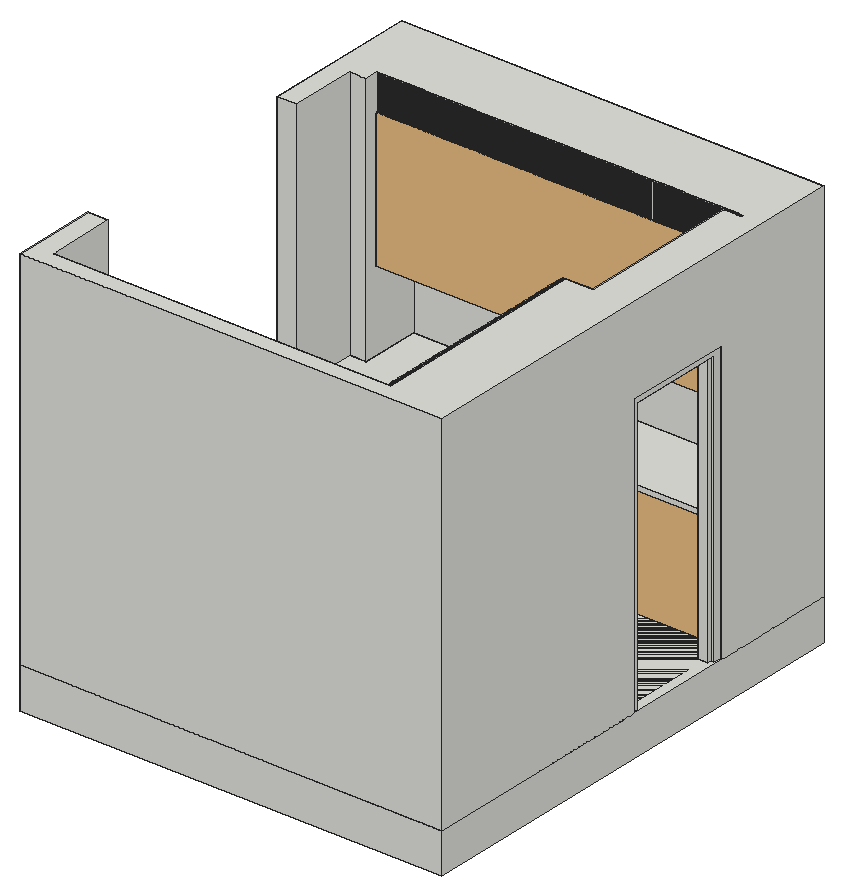
# SketchUp Ruby script. Lengths in millimetres.
U = 1.mm
M = Sketchup.active_model
def pt(a) = Geom::Point3d.new(a.map { |v| v * U })
def face(e, loops, mat)
  f = e.add_face(loops[0].map { |a| pt(a) })
  loops[1..].each { |l| e.add_face(l.map { |a| pt(a) }).erase! }
  f.material = f.back_material = mat if mat
  f
end
# faces: each face lists its corners as indices into pts; further lists are holes
def faces(e, pts, list, mat = nil) = list.each { |f| face(e, (f[0].is_a?(Array) ? f : [f]).map { |l| l.map { |i| pts[i] } }, mat) }
# xy, xz, yz: faces in a plane at the given z, y or x. An outline is a flat list of corners, or four numbers for a rectangle; further outlines are holes
def ring(l) = l.size == 4 ? [[l[0], l[1]], [l[2], l[1]], [l[2], l[3]], [l[0], l[3]]] : l.each_slice(2).to_a
def flat(e, list, mat, &to3) = list.each { |f| face(e, (f[0].is_a?(Array) ? f : [f]).map { |l| ring(l).map { |u, v| to3.(u, v) } }, mat) }
def xy(e, z, list, mat = nil) = flat(e, list, mat) { |x, y| [x, y, z] }
def xz(e, y, list, mat = nil) = flat(e, list, mat) { |x, z| [x, y, z] }
def yz(e, x, list, mat = nil) = flat(e, list, mat) { |y, z| [x, y, z] }
def lines(e, pts, list) = list.each { |a, b| e.add_line(pt(pts[a]), pt(pts[b])) }
# prism: a flat outline (further loops are holes) pulled along v
def prism(e, loops, v, mat = nil)
  f = face(e, loops, mat); d = Geom::Vector3d.new(v.map { |x| x * U })
  f.pushpull(f.normal.samedirection?(d) ? d.length : -d.length)
end
def box(e, o, s, mat = nil) = prism(e, [[o, [o[0] + s[0], o[1], o[2]], [o[0] + s[0], o[1] + s[1], o[2]], [o[0], o[1] + s[1], o[2]]]], [0, 0, s[2]], mat)
def at(x, y, z, deg = 0) = Geom::Transformation.translation(pt([x, y, z])) * Geom::Transformation.rotation(ORIGIN, Z_AXIS, deg.degrees)
def axes(o, x, y, z) = Geom::Transformation.new([*x, 0, *y, 0, *z, 0, *pt(o).to_a, 1])
def part(name) = M.definitions.add(name)
# library, detail: a bought-in or finely detailed component or shape, given as its bounding box
def library(name, o, s) = part(name).tap { |d| box(d.entities, o, s) }
def detail(e, o, s) = box(e.add_group.entities, o, s)
def put(e, d, t, mat = nil) = e.add_instance(d, t).tap { |i| i.material = mat if mat }
def group(e, t, mat = nil) = e.add_group.tap { |g| g.transformation = t; g.material = mat if mat }.entities
root = M.entities
c1 = part("skp9A08")
detail(c1.entities,[955.4,-577.1,1130.3],[195.9,193,77.6])
c2 = part("Memento Mori 2 - Living Room and Bedroom JhonyHebert")
put(c2.entities,c1,at(1865.8,0,3866.9))
c3 = part("Basket")
put(c3.entities,c2,at(22136,105695.5,0))
c4 = library("Group\#3",[-125,0,0],[2845,600,820])
c5 = library("Group\#4",[0,-350,0],[2720,368,1030])
c6 = part("Group5\#1")
xy(c6.entities,0,[[-410,-1050,-410,1050,410,1050,410,-1050,360,-1050,360,1000,-360,1000,-360,-1050]])
xy(c6.entities,25,[[-360,-1050,-360,1000,360,1000,360,-1050,335,-1050,335,975,-335,975,-335,-1050]])
xy(c6.entities,100,[[-360,-1050,-335,-1050,-335,975,335,975,335,-1050,360,-1050,360,1000,-360,1000]])
xy(c6.entities,125,[[-410,-1050,-360,-1050,-360,1000,360,1000,360,-1050,410,-1050,410,1050,-410,1050]])
xz(c6.entities,-1050,[[-410,0,-360,125],[360,0,410,125],[-360,25,-335,100],[335,25,360,100]])
xz(c6.entities,975,[[-335,25,335,100]])
xz(c6.entities,1000,[[-360,0,360,25],[-360,100,360,125]])
xz(c6.entities,1050,[[-410,0,410,125]])
yz(c6.entities,-410,[[-1050,0,1050,125]])
yz(c6.entities,-360,[[-1050,0,1000,25],[-1050,100,1000,125]])
yz(c6.entities,-335,[[-1050,25,975,100]])
yz(c6.entities,335,[[-1050,25,975,100]])
yz(c6.entities,360,[[-1050,0,1000,25],[-1050,100,1000,125]])
yz(c6.entities,410,[[-1050,0,1050,125]])
c7 = library("Group\#5",[-350,0,0],[350,1630,1030])
c8 = part("Group\#6")
box(c8.entities,[-20,0,0],[20,15.2,260])
xy(root,0,[[0,0,0,634,148,634,148,124,2993,124,2993,1784,3148,1784,3148,0],[148,124,2993,124,2993,1784,3070.5,1784,3070.5,2604,2993,2604,2993,3324,273,3324,273,2884,148,2884,148,2394,0,2394,0,634,148,634],[3070.5,1784,3148,2604],[0,2394,0,3553,3148,3553,3148,2604,2993,2604,2993,3324,273,3324,273,2884,148,2884,148,2394]])
xy(root,100,[[2393,124,2993,724],[2393,724,2993,774],[2393,774,2993,1304],[2393,1304,2993,1754]])
xy(root,125,[[2393,1329,2993,1729]])
xy(root,451,[[2393,124,2411,724],[2393,774,2411,1304]])
xy(root,469,[[2393,124,2411,724],[2393,774,2411,1304]])
xy(root,790,[[2393,124,2993,724],[2393,774,2411,1304]])
xy(root,795,[[2393,1329,2993,1729]])
xy(root,820,[[2393,724,2993,774],[2411,774,2993,1304],[2393,1304,2993,1754]])
xy(root,2100,[[2993,1784,3070.5,2604],[3070.5,1784,3148,2604]])
xy(root,2490,[[2663,124,2993,1754],[288,2974,303,2986],[308,2974,323,2986],[328,2974,343,2986],[348,2974,363,2986],
  [368,2974,383,2986],[388,2974,403,2986],[408,2974,423,2986],[428,2974,443,2986],[448,2974,463,2986],
  [468,2974,483,2986],[488,2974,503,2986],[508,2974,523,2986],[528,2974,543,2986],[548,2974,563,2986],
  [568,2974,583,2986],[588,2974,603,2986],[608,2974,623,2986],[628,2974,643,2986],[648,2974,663,2986],
  [668,2974,683,2986],[688,2974,703,2986],[708,2974,723,2986],[728,2974,743,2986],[748,2974,763,2986],
  [768,2974,783,2986],[788,2974,803,2986],[808,2974,823,2986],[828,2974,843,2986],[848,2974,863,2986],
  [868,2974,883,2986],[888,2974,903,2986],[908,2974,923,2986],[928,2974,943,2986],[948,2974,963,2986],
  [968,2974,983,2986],[988,2974,1003,2986],[1008,2974,1023,2986],[1028,2974,1043,2986],[1048,2974,1063,2986],
  [1068,2974,1083,2986],[1088,2974,1103,2986],[1108,2974,1123,2986],[1128,2974,1143,2986],[1148,2974,1163,2986],
  [1168,2974,1183,2986],[1188,2974,1203,2986],[1208,2974,1223,2986],[1228,2974,1243,2986],[1248,2974,1263,2986],
  [1268,2974,1283,2986],[1288,2974,1303,2986],[1308,2974,1323,2986],[1328,2974,1343,2986],[1348,2974,1363,2986],
  [1368,2974,1383,2986],[1388,2974,1403,2986],[1408,2974,1423,2986],[1428,2974,1443,2986],[1448,2974,1463,2986],
  [1468,2974,1483,2986],[1488,2974,1503,2986],[1508,2974,1523,2986],[1528,2974,1543,2986],[1548,2974,1563,2986],
  [1568,2974,1583,2986],[1588,2974,1603,2986],[1608,2974,1623,2986],[1628,2974,1643,2986],[1648,2974,1663,2986],
  [1668,2974,1683,2986],[1688,2974,1703,2986],[1708,2974,1723,2986],[1728,2974,1743,2986],[1748,2974,1763,2986],
  [1768,2974,1783,2986],[1788,2974,1803,2986],[1808,2974,1823,2986],[1828,2974,1843,2986],[1848,2974,1863,2986],
  [1868,2974,1883,2986],[1888,2974,1903,2986],[1908,2974,1923,2986],[1928,2974,1943,2986],[1948,2974,1963,2986],
  [1968,2974,1983,2986],[1988,2974,2003,2986],[2008,2974,2023,2986],[2028,2974,2043,2986],[2048,2974,2063,2986],
  [2068,2974,2083,2986],[2088,2974,2103,2986],[2108,2974,2123,2986],[2128,2974,2143,2986],[2148,2974,2163,2986],
  [2168,2974,2183,2986],[2188,2974,2203,2986],[2208,2974,2223,2986],[2228,2974,2243,2986],[2248,2974,2263,2986],
  [2268,2974,2283,2986],[2288,2974,2303,2986],[2308,2974,2323,2986],[2328,2974,2343,2986],[2348,2974,2363,2986],
  [2368,2974,2383,2986],[2388,2974,2403,2986],[2408,2974,2423,2986],[2428,2974,2443,2986],[2448,2974,2463,2986],
  [2468,2974,2483,2986],[2488,2974,2503,2986],[2508,2974,2523,2986],[2528,2974,2543,2986],[2548,2974,2563,2986],
  [2568,2974,2583,2986],[2588,2974,2603,2986],[2608,2974,2623,2986],[2628,2974,2643,2986],[2648,2974,2663,2986],
  [2668,2974,2683,2986],[2688,2974,2703,2986],[2708,2974,2723,2986],[2728,2974,2743,2986],[2748,2974,2763,2986],
  [2768,2974,2783,2986],[2788,2974,2803,2986],[2808,2974,2823,2986],[2828,2974,2843,2986],[2848,2974,2863,2986],
  [2868,2974,2883,2986],[2888,2974,2903,2986],[2908,2974,2923,2986],[2928,2974,2943,2986],[2948,2974,2963,2986],
  [2968,2974,2983,2986],[2988,2974,3003,2986],[273,2986,309.5,3324],[309.5,2986,316.5,3324],[316.5,2986,1149.5,3324],
  [1149.5,2986,1156.5,3324],[1156.5,2986,1729.5,3324],[1729.5,2986,2376.5,3324],[2376.5,2986,2949.5,3324],[2949.5,2986,2956.5,3324],
  [2956.5,2986,2993,3324]])
xy(root,2600,[[2868,1754,2993,2986]])
xy(root,2750,[[[0,0,3148,0,3148,3553,0,3553,0,2394,148,2394,148,2884,273,2884,273,2986,2883,2986,2883,2974,2868,2974,2868,1754,2663,1754,2663,124,148,124,148,634,0,634],[2908,2974,2923,2986],[2928,2974,2943,2986],[2988,2974,3003,2986],[2968,2974,2983,2986],[2888,2974,2903,2986],[2948,2974,2963,2986]],[288,2974,303,2986],[308,2974,323,2986],[328,2974,343,2986],[348,2974,363,2986],
  [368,2974,383,2986],[388,2974,403,2986],[408,2974,423,2986],[428,2974,443,2986],[448,2974,463,2986],
  [468,2974,483,2986],[488,2974,503,2986],[508,2974,523,2986],[528,2974,543,2986],[548,2974,563,2986],
  [568,2974,583,2986],[588,2974,603,2986],[608,2974,623,2986],[628,2974,643,2986],[648,2974,663,2986],
  [668,2974,683,2986],[688,2974,703,2986],[708,2974,723,2986],[728,2974,743,2986],[748,2974,763,2986],
  [768,2974,783,2986],[788,2974,803,2986],[808,2974,823,2986],[828,2974,843,2986],[848,2974,863,2986],
  [868,2974,883,2986],[888,2974,903,2986],[908,2974,923,2986],[928,2974,943,2986],[948,2974,963,2986],
  [968,2974,983,2986],[988,2974,1003,2986],[1008,2974,1023,2986],[1028,2974,1043,2986],[1048,2974,1063,2986],
  [1068,2974,1083,2986],[1088,2974,1103,2986],[1108,2974,1123,2986],[1128,2974,1143,2986],[1148,2974,1163,2986],
  [1168,2974,1183,2986],[1188,2974,1203,2986],[1208,2974,1223,2986],[1228,2974,1243,2986],[1248,2974,1263,2986],
  [1268,2974,1283,2986],[1288,2974,1303,2986],[1308,2974,1323,2986],[1328,2974,1343,2986],[1348,2974,1363,2986],
  [1368,2974,1383,2986],[1388,2974,1403,2986],[1408,2974,1423,2986],[1428,2974,1443,2986],[1448,2974,1463,2986],
  [1468,2974,1483,2986],[1488,2974,1503,2986],[1508,2974,1523,2986],[1528,2974,1543,2986],[1548,2974,1563,2986],
  [1568,2974,1583,2986],[1588,2974,1603,2986],[1608,2974,1623,2986],[1628,2974,1643,2986],[1648,2974,1663,2986],
  [1668,2974,1683,2986],[1688,2974,1703,2986],[1708,2974,1723,2986],[1728,2974,1743,2986],[1748,2974,1763,2986],
  [1768,2974,1783,2986],[1788,2974,1803,2986],[1808,2974,1823,2986],[1828,2974,1843,2986],[1848,2974,1863,2986],
  [1868,2974,1883,2986],[1888,2974,1903,2986],[1908,2974,1923,2986],[1928,2974,1943,2986],[1948,2974,1963,2986],
  [1968,2974,1983,2986],[1988,2974,2003,2986],[2008,2974,2023,2986],[2028,2974,2043,2986],[2048,2974,2063,2986],
  [2068,2974,2083,2986],[2088,2974,2103,2986],[2108,2974,2123,2986],[2128,2974,2143,2986],[2148,2974,2163,2986],
  [2168,2974,2183,2986],[2188,2974,2203,2986],[2208,2974,2223,2986],[2228,2974,2243,2986],[2248,2974,2263,2986],
  [2268,2974,2283,2986],[2288,2974,2303,2986],[2308,2974,2323,2986],[2328,2974,2343,2986],[2348,2974,2363,2986],
  [2368,2974,2383,2986],[2388,2974,2403,2986],[2408,2974,2423,2986],[2428,2974,2443,2986],[2448,2974,2463,2986],
  [2468,2974,2483,2986],[2488,2974,2503,2986],[2508,2974,2523,2986],[2528,2974,2543,2986],[2548,2974,2563,2986],
  [2568,2974,2583,2986],[2588,2974,2603,2986],[2608,2974,2623,2986],[2628,2974,2643,2986],[2648,2974,2663,2986],
  [2668,2974,2683,2986],[2688,2974,2703,2986],[2708,2974,2723,2986],[2728,2974,2743,2986],[2748,2974,2763,2986],
  [2768,2974,2783,2986],[2788,2974,2803,2986],[2808,2974,2823,2986],[2828,2974,2843,2986],[2848,2974,2863,2986],
  [2868,2974,2883,2986],[2888,2974,2903,2986],[2908,2974,2923,2986],[2928,2974,2943,2986],[2948,2974,2963,2986],
  [2968,2974,2983,2986],[2988,2974,3003,2986]])
xz(root,0,[[0,0,3148,2750]])
xz(root,124,[[148,0,148,2750,2663,2750,2663,2490,2993,2490,2993,790,2393,790,2393,469,2411,469,2411,451,2393,451,2393,100,2993,100,2993,0],[2393,100,2393,451,2411,451,2411,469,2393,469,2393,790,2993,790,2993,100]])
xz(root,634,[[0,0,148,2750]])
xz(root,724,[[2393,451,2411,469],[2393,790,2993,820]])
xz(root,774,[[2393,451,2411,469],[2393,790,2411,820]])
xz(root,1304,[[2393,451,2411,460],[2393,460,2411,469],[2393,790,2411,820]])
xz(root,1329,[[2393,125,2993,795]])
xz(root,1729,[[2393,125,2993,795]])
xz(root,1754,[[2393,100,2993,820],[2663,2490,2663,2750,2868,2750,2868,2600,2993,2600,2993,2490]])
xz(root,1784,[[2993,0,3070.5,2100],[3070.5,0,3148,2100]])
xz(root,2394,[[0,0,148,2750]])
xz(root,2604,[[2993,0,3070.5,2100],[3070.5,0,3148,2100]])
xz(root,2884,[[148,0,273,860],[148,860,273,2750]])
xz(root,2974,[[288,2490,303,2750],[308,2490,323,2750],[328,2490,343,2750],[348,2490,363,2750],[368,2490,383,2750],
  [388,2490,403,2750],[408,2490,423,2750],[428,2490,443,2750],[448,2490,463,2750],[468,2490,483,2750],
  [488,2490,503,2750],[508,2490,523,2750],[528,2490,543,2750],[548,2490,563,2750],[568,2490,583,2750],
  [588,2490,603,2750],[608,2490,623,2750],[628,2490,643,2750],[648,2490,663,2750],[668,2490,683,2750],
  [688,2490,703,2750],[708,2490,723,2750],[728,2490,743,2750],[748,2490,763,2750],[768,2490,783,2750],
  [788,2490,803,2750],[808,2490,823,2750],[828,2490,843,2750],[848,2490,863,2750],[868,2490,883,2750],
  [888,2490,903,2750],[908,2490,923,2750],[928,2490,943,2750],[948,2490,963,2750],[968,2490,983,2750],
  [988,2490,1003,2750],[1008,2490,1023,2750],[1028,2490,1043,2750],[1048,2490,1063,2750],[1068,2490,1083,2750],
  [1088,2490,1103,2750],[1108,2490,1123,2750],[1128,2490,1143,2750],[1148,2490,1163,2750],[1168,2490,1183,2750],
  [1188,2490,1203,2750],[1208,2490,1223,2750],[1228,2490,1243,2750],[1248,2490,1263,2750],[1268,2490,1283,2750],
  [1288,2490,1303,2750],[1308,2490,1323,2750],[1328,2490,1343,2750],[1348,2490,1363,2750],[1368,2490,1383,2750],
  [1388,2490,1403,2750],[1408,2490,1423,2750],[1428,2490,1443,2750],[1448,2490,1463,2750],[1468,2490,1483,2750],
  [1488,2490,1503,2750],[1508,2490,1523,2750],[1528,2490,1543,2750],[1548,2490,1563,2750],[1568,2490,1583,2750],
  [1588,2490,1603,2750],[1608,2490,1623,2750],[1628,2490,1643,2750],[1648,2490,1663,2750],[1668,2490,1683,2750],
  [1688,2490,1703,2750],[1708,2490,1723,2750],[1728,2490,1743,2750],[1748,2490,1763,2750],[1768,2490,1783,2750],
  [1788,2490,1803,2750],[1808,2490,1823,2750],[1828,2490,1843,2750],[1848,2490,1863,2750],[1868,2490,1883,2750],
  [1888,2490,1903,2750],[1908,2490,1923,2750],[1928,2490,1943,2750],[1948,2490,1963,2750],[1968,2490,1983,2750],
  [1988,2490,2003,2750],[2008,2490,2023,2750],[2028,2490,2043,2750],[2048,2490,2063,2750],[2068,2490,2083,2750],
  [2088,2490,2103,2750],[2108,2490,2123,2750],[2128,2490,2143,2750],[2148,2490,2163,2750],[2168,2490,2183,2750],
  [2188,2490,2203,2750],[2208,2490,2223,2750],[2228,2490,2243,2750],[2248,2490,2263,2750],[2268,2490,2283,2750],
  [2288,2490,2303,2750],[2308,2490,2323,2750],[2328,2490,2343,2750],[2348,2490,2363,2750],[2368,2490,2383,2750],
  [2388,2490,2403,2750],[2408,2490,2423,2750],[2428,2490,2443,2750],[2448,2490,2463,2750],[2468,2490,2483,2750],
  [2488,2490,2503,2750],[2508,2490,2523,2750],[2528,2490,2543,2750],[2548,2490,2563,2750],[2568,2490,2583,2750],
  [2588,2490,2603,2750],[2608,2490,2623,2750],[2628,2490,2643,2750],[2648,2490,2663,2750],[2668,2490,2683,2750],
  [2688,2490,2703,2750],[2708,2490,2723,2750],[2728,2490,2743,2750],[2748,2490,2763,2750],[2768,2490,2783,2750],
  [2788,2490,2803,2750],[2808,2490,2823,2750],[2828,2490,2843,2750],[2848,2490,2863,2750],[2868,2490,2883,2750],
  [2888,2490,2903,2750],[2908,2490,2923,2750],[2928,2490,2943,2750],[2948,2490,2963,2750],[2968,2490,2983,2750],
  [2988,2490,3003,2750]])
xz(root,2986,[[273,2490,288,2750],[288,2490,303,2750],[303,2490,308,2750],[308,2490,323,2750],[323,2490,328,2750],
  [328,2490,343,2750],[343,2490,348,2750],[348,2490,363,2750],[363,2490,368,2750],[368,2490,383,2750],
  [383,2490,388,2750],[388,2490,403,2750],[403,2490,408,2750],[408,2490,423,2750],[423,2490,428,2750],
  [428,2490,443,2750],[443,2490,448,2750],[448,2490,463,2750],[463,2490,468,2750],[468,2490,483,2750],
  [483,2490,488,2750],[488,2490,503,2750],[503,2490,508,2750],[508,2490,523,2750],[523,2490,528,2750],
  [528,2490,543,2750],[543,2490,548,2750],[548,2490,563,2750],[563,2490,568,2750],[568,2490,583,2750],
  [583,2490,588,2750],[588,2490,603,2750],[603,2490,608,2750],[608,2490,623,2750],[623,2490,628,2750],
  [628,2490,643,2750],[643,2490,648,2750],[648,2490,663,2750],[663,2490,668,2750],[668,2490,683,2750],
  [683,2490,688,2750],[688,2490,703,2750],[703,2490,708,2750],[708,2490,723,2750],[723,2490,728,2750],
  [728,2490,743,2750],[743,2490,748,2750],[748,2490,763,2750],[763,2490,768,2750],[768,2490,783,2750],
  [783,2490,788,2750],[788,2490,803,2750],[803,2490,808,2750],[808,2490,823,2750],[823,2490,828,2750],
  [828,2490,843,2750],[843,2490,848,2750],[848,2490,863,2750],[863,2490,868,2750],[868,2490,883,2750],
  [883,2490,888,2750],[888,2490,903,2750],[903,2490,908,2750],[908,2490,923,2750],[923,2490,928,2750],
  [928,2490,943,2750],[943,2490,948,2750],[948,2490,963,2750],[963,2490,968,2750],[968,2490,983,2750],
  [983,2490,988,2750],[988,2490,1003,2750],[1003,2490,1008,2750],[1008,2490,1023,2750],[1023,2490,1028,2750],
  [1028,2490,1043,2750],[1043,2490,1048,2750],[1048,2490,1063,2750],[1063,2490,1068,2750],[1068,2490,1083,2750],
  [1083,2490,1088,2750],[1088,2490,1103,2750],[1103,2490,1108,2750],[1108,2490,1123,2750],[1123,2490,1128,2750],
  [1128,2490,1143,2750],[1143,2490,1148,2750],[1148,2490,1163,2750],[1163,2490,1168,2750],[1168,2490,1183,2750],
  [1183,2490,1188,2750],[1188,2490,1203,2750],[1203,2490,1208,2750],[1208,2490,1223,2750],[1223,2490,1228,2750],
  [1228,2490,1243,2750],[1243,2490,1248,2750],[1248,2490,1263,2750],[1263,2490,1268,2750],[1268,2490,1283,2750],
  [1283,2490,1288,2750],[1288,2490,1303,2750],[1303,2490,1308,2750],[1308,2490,1323,2750],[1323,2490,1328,2750],
  [1328,2490,1343,2750],[1343,2490,1348,2750],[1348,2490,1363,2750],[1363,2490,1368,2750],[1368,2490,1383,2750],
  [1383,2490,1388,2750],[1388,2490,1403,2750],[1403,2490,1408,2750],[1408,2490,1423,2750],[1423,2490,1428,2750],
  [1428,2490,1443,2750],[1443,2490,1448,2750],[1448,2490,1463,2750],[1463,2490,1468,2750],[1468,2490,1483,2750],
  [1483,2490,1488,2750],[1488,2490,1503,2750],[1503,2490,1508,2750],[1508,2490,1523,2750],[1523,2490,1528,2750],
  [1528,2490,1543,2750],[1543,2490,1548,2750],[1548,2490,1563,2750],[1563,2490,1568,2750],[1568,2490,1583,2750],
  [1583,2490,1588,2750],[1588,2490,1603,2750],[1603,2490,1608,2750],[1608,2490,1623,2750],[1623,2490,1628,2750],
  [1628,2490,1643,2750],[1643,2490,1648,2750],[1648,2490,1663,2750],[1663,2490,1668,2750],[1668,2490,1683,2750],
  [1683,2490,1688,2750],[1688,2490,1703,2750],[1703,2490,1708,2750],[1708,2490,1723,2750],[1723,2490,1728,2750],
  [1728,2490,1743,2750],[1743,2490,1748,2750],[1748,2490,1763,2750],[1763,2490,1768,2750],[1768,2490,1783,2750],
  [1783,2490,1788,2750],[1788,2490,1803,2750],[1803,2490,1808,2750],[1808,2490,1823,2750],[1823,2490,1828,2750],
  [1828,2490,1843,2750],[1843,2490,1848,2750],[1848,2490,1863,2750],[1863,2490,1868,2750],[1868,2490,1883,2750],
  [1883,2490,1888,2750],[1888,2490,1903,2750],[1903,2490,1908,2750],[1908,2490,1923,2750],[1923,2490,1928,2750],
  [1928,2490,1943,2750],[1943,2490,1948,2750],[1948,2490,1963,2750],[1963,2490,1968,2750],[1968,2490,1983,2750],
  [1983,2490,1988,2750],[1988,2490,2003,2750],[2003,2490,2008,2750],[2008,2490,2023,2750],[2023,2490,2028,2750],
  [2028,2490,2043,2750],[2043,2490,2048,2750],[2048,2490,2063,2750],[2063,2490,2068,2750],[2068,2490,2083,2750],
  [2083,2490,2088,2750],[2088,2490,2103,2750],[2103,2490,2108,2750],[2108,2490,2123,2750],[2123,2490,2128,2750],
  [2128,2490,2143,2750],[2143,2490,2148,2750],[2148,2490,2163,2750],[2163,2490,2168,2750],[2168,2490,2183,2750],
  [2183,2490,2188,2750],[2188,2490,2203,2750],[2203,2490,2208,2750],[2208,2490,2223,2750],[2223,2490,2228,2750],
  [2228,2490,2243,2750],[2243,2490,2248,2750],[2248,2490,2263,2750],[2263,2490,2268,2750],[2268,2490,2283,2750],
  [2283,2490,2288,2750],[2288,2490,2303,2750],[2303,2490,2308,2750],[2308,2490,2323,2750],[2323,2490,2328,2750],
  [2328,2490,2343,2750],[2343,2490,2348,2750],[2348,2490,2363,2750],[2363,2490,2368,2750],[2368,2490,2383,2750],
  [2383,2490,2388,2750],[2388,2490,2403,2750],[2403,2490,2408,2750],[2408,2490,2423,2750],[2423,2490,2428,2750],
  [2428,2490,2443,2750],[2443,2490,2448,2750],[2448,2490,2463,2750],[2463,2490,2468,2750],[2468,2490,2483,2750],
  [2483,2490,2488,2750],[2488,2490,2503,2750],[2503,2490,2508,2750],[2508,2490,2523,2750],[2523,2490,2528,2750],
  [2528,2490,2543,2750],[2543,2490,2548,2750],[2548,2490,2563,2750],[2563,2490,2568,2750],[2568,2490,2583,2750],
  [2583,2490,2588,2750],[2588,2490,2603,2750],[2603,2490,2608,2750],[2608,2490,2623,2750],[2623,2490,2628,2750],
  [2628,2490,2643,2750],[2643,2490,2648,2750],[2648,2490,2663,2750],[2663,2490,2668,2750],[2668,2490,2683,2750],
  [2683,2490,2688,2750],[2688,2490,2703,2750],[2703,2490,2708,2750],[2708,2490,2723,2750],[2723,2490,2728,2750],
  [2728,2490,2743,2750],[2743,2490,2748,2750],[2748,2490,2763,2750],[2763,2490,2768,2750],[2768,2490,2783,2750],
  [2783,2490,2788,2750],[2788,2490,2803,2750],[2803,2490,2808,2750],[2808,2490,2823,2750],[2823,2490,2828,2750],
  [2828,2490,2843,2750],[2843,2490,2848,2750],[2848,2490,2863,2750],[2863,2490,2868,2750],[2868,2490,2883,2600],
  [2883,2490,2888,2600],[2888,2490,2903,2600],[2903,2490,2908,2600],[2908,2490,2923,2600],[2923,2490,2928,2600],
  [2928,2490,2943,2600],[2943,2490,2948,2600],[2948,2490,2963,2600],[2963,2490,2968,2600],[2968,2490,2983,2600],
  [2983,2490,2988,2600],[2988,2490,2993,2600],[2993,2490,2993,2600,2988,2600,2988,2750,3003,2750,3003,2490],[2868,2600,2883,2750],[2888,2600,2903,2750],
  [2908,2600,2923,2750],[2928,2600,2943,2750],[2948,2600,2963,2750],[2968,2600,2983,2750]])
xz(root,3324,[[273,0,2993,860],[273,860,2993,860,2993,1460,2956.5,1460,2956.5,2490,2949.5,2490,2949.5,1460,2376.5,1460,2376.5,2490,1729.5,2490,1729.5,1460,1156.5,1460,1156.5,2490,1149.5,2490,1149.5,1460,316.5,1460,316.5,2490,309.5,2490,309.5,1460,273,1460],[273,1460,309.5,2490],[316.5,1460,1149.5,2490],[1156.5,1460,1729.5,2490],
  [2376.5,1460,2949.5,2490],[2956.5,1460,2993,2490],[2993,1460,2993.5,2490]])
xz(root,3553,[[0,0,3148,2750]])
yz(root,0,[[0,0,634,2750],[2394,0,3553,2750]])
yz(root,148,[[124,0,634,2750],[2394,0,2884,2750]])
yz(root,273,[[2884,0,3324,860],[2884,860,3324,860,3324,2490,2986,2490,2986,2750,2884,2750]])
yz(root,288,[[2974,2490,2986,2750]])
yz(root,303,[[2974,2490,2986,2750]])
yz(root,308,[[2974,2490,2986,2750]])
yz(root,323,[[2974,2490,2986,2750]])
yz(root,328,[[2974,2490,2986,2750]])
yz(root,343,[[2974,2490,2986,2750]])
yz(root,348,[[2974,2490,2986,2750]])
yz(root,363,[[2974,2490,2986,2750]])
yz(root,368,[[2974,2490,2986,2750]])
yz(root,383,[[2974,2490,2986,2750]])
yz(root,388,[[2974,2490,2986,2750]])
yz(root,403,[[2974,2490,2986,2750]])
yz(root,408,[[2974,2490,2986,2750]])
yz(root,423,[[2974,2490,2986,2750]])
yz(root,428,[[2974,2490,2986,2750]])
yz(root,443,[[2974,2490,2986,2750]])
yz(root,448,[[2974,2490,2986,2750]])
yz(root,463,[[2974,2490,2986,2750]])
yz(root,468,[[2974,2490,2986,2750]])
yz(root,483,[[2974,2490,2986,2750]])
yz(root,488,[[2974,2490,2986,2750]])
yz(root,503,[[2974,2490,2986,2750]])
yz(root,508,[[2974,2490,2986,2750]])
yz(root,523,[[2974,2490,2986,2750]])
yz(root,528,[[2974,2490,2986,2750]])
yz(root,543,[[2974,2490,2986,2750]])
yz(root,548,[[2974,2490,2986,2750]])
yz(root,563,[[2974,2490,2986,2750]])
yz(root,568,[[2974,2490,2986,2750]])
yz(root,583,[[2974,2490,2986,2750]])
yz(root,588,[[2974,2490,2986,2750]])
yz(root,603,[[2974,2490,2986,2750]])
yz(root,608,[[2974,2490,2986,2750]])
yz(root,623,[[2974,2490,2986,2750]])
yz(root,628,[[2974,2490,2986,2750]])
yz(root,643,[[2974,2490,2986,2750]])
yz(root,648,[[2974,2490,2986,2750]])
yz(root,663,[[2974,2490,2986,2750]])
yz(root,668,[[2974,2490,2986,2750]])
yz(root,683,[[2974,2490,2986,2750]])
yz(root,688,[[2974,2490,2986,2750]])
yz(root,703,[[2974,2490,2986,2750]])
yz(root,708,[[2974,2490,2986,2750]])
yz(root,723,[[2974,2490,2986,2750]])
yz(root,728,[[2974,2490,2986,2750]])
yz(root,743,[[2974,2490,2986,2750]])
yz(root,748,[[2974,2490,2986,2750]])
yz(root,763,[[2974,2490,2986,2750]])
yz(root,768,[[2974,2490,2986,2750]])
yz(root,783,[[2974,2490,2986,2750]])
yz(root,788,[[2974,2490,2986,2750]])
yz(root,803,[[2974,2490,2986,2750]])
yz(root,808,[[2974,2490,2986,2750]])
yz(root,823,[[2974,2490,2986,2750]])
yz(root,828,[[2974,2490,2986,2750]])
yz(root,843,[[2974,2490,2986,2750]])
yz(root,848,[[2974,2490,2986,2750]])
yz(root,863,[[2974,2490,2986,2750]])
yz(root,868,[[2974,2490,2986,2750]])
yz(root,883,[[2974,2490,2986,2750]])
yz(root,888,[[2974,2490,2986,2750]])
yz(root,903,[[2974,2490,2986,2750]])
yz(root,908,[[2974,2490,2986,2750]])
yz(root,923,[[2974,2490,2986,2750]])
yz(root,928,[[2974,2490,2986,2750]])
yz(root,943,[[2974,2490,2986,2750]])
yz(root,948,[[2974,2490,2986,2750]])
yz(root,963,[[2974,2490,2986,2750]])
yz(root,968,[[2974,2490,2986,2750]])
yz(root,983,[[2974,2490,2986,2750]])
yz(root,988,[[2974,2490,2986,2750]])
yz(root,1003,[[2974,2490,2986,2750]])
yz(root,1008,[[2974,2490,2986,2750]])
yz(root,1023,[[2974,2490,2986,2750]])
yz(root,1028,[[2974,2490,2986,2750]])
yz(root,1043,[[2974,2490,2986,2750]])
yz(root,1048,[[2974,2490,2986,2750]])
yz(root,1063,[[2974,2490,2986,2750]])
yz(root,1068,[[2974,2490,2986,2750]])
yz(root,1083,[[2974,2490,2986,2750]])
yz(root,1088,[[2974,2490,2986,2750]])
yz(root,1103,[[2974,2490,2986,2750]])
yz(root,1108,[[2974,2490,2986,2750]])
yz(root,1123,[[2974,2490,2986,2750]])
yz(root,1128,[[2974,2490,2986,2750]])
yz(root,1143,[[2974,2490,2986,2750]])
yz(root,1148,[[2974,2490,2986,2750]])
yz(root,1163,[[2974,2490,2986,2750]])
yz(root,1168,[[2974,2490,2986,2750]])
yz(root,1183,[[2974,2490,2986,2750]])
yz(root,1188,[[2974,2490,2986,2750]])
yz(root,1203,[[2974,2490,2986,2750]])
yz(root,1208,[[2974,2490,2986,2750]])
yz(root,1223,[[2974,2490,2986,2750]])
yz(root,1228,[[2974,2490,2986,2750]])
yz(root,1243,[[2974,2490,2986,2750]])
yz(root,1248,[[2974,2490,2986,2750]])
yz(root,1263,[[2974,2490,2986,2750]])
yz(root,1268,[[2974,2490,2986,2750]])
yz(root,1283,[[2974,2490,2986,2750]])
yz(root,1288,[[2974,2490,2986,2750]])
yz(root,1303,[[2974,2490,2986,2750]])
yz(root,1308,[[2974,2490,2986,2750]])
yz(root,1323,[[2974,2490,2986,2750]])
yz(root,1328,[[2974,2490,2986,2750]])
yz(root,1343,[[2974,2490,2986,2750]])
yz(root,1348,[[2974,2490,2986,2750]])
yz(root,1363,[[2974,2490,2986,2750]])
yz(root,1368,[[2974,2490,2986,2750]])
yz(root,1383,[[2974,2490,2986,2750]])
yz(root,1388,[[2974,2490,2986,2750]])
yz(root,1403,[[2974,2490,2986,2750]])
yz(root,1408,[[2974,2490,2986,2750]])
yz(root,1423,[[2974,2490,2986,2750]])
yz(root,1428,[[2974,2490,2986,2750]])
yz(root,1443,[[2974,2490,2986,2750]])
yz(root,1448,[[2974,2490,2986,2750]])
yz(root,1463,[[2974,2490,2986,2750]])
yz(root,1468,[[2974,2490,2986,2750]])
yz(root,1483,[[2974,2490,2986,2750]])
yz(root,1488,[[2974,2490,2986,2750]])
yz(root,1503,[[2974,2490,2986,2750]])
yz(root,1508,[[2974,2490,2986,2750]])
yz(root,1523,[[2974,2490,2986,2750]])
yz(root,1528,[[2974,2490,2986,2750]])
yz(root,1543,[[2974,2490,2986,2750]])
yz(root,1548,[[2974,2490,2986,2750]])
yz(root,1563,[[2974,2490,2986,2750]])
yz(root,1568,[[2974,2490,2986,2750]])
yz(root,1583,[[2974,2490,2986,2750]])
yz(root,1588,[[2974,2490,2986,2750]])
yz(root,1603,[[2974,2490,2986,2750]])
yz(root,1608,[[2974,2490,2986,2750]])
yz(root,1623,[[2974,2490,2986,2750]])
yz(root,1628,[[2974,2490,2986,2750]])
yz(root,1643,[[2974,2490,2986,2750]])
yz(root,1648,[[2974,2490,2986,2750]])
yz(root,1663,[[2974,2490,2986,2750]])
yz(root,1668,[[2974,2490,2986,2750]])
yz(root,1683,[[2974,2490,2986,2750]])
yz(root,1688,[[2974,2490,2986,2750]])
yz(root,1703,[[2974,2490,2986,2750]])
yz(root,1708,[[2974,2490,2986,2750]])
yz(root,1723,[[2974,2490,2986,2750]])
yz(root,1728,[[2974,2490,2986,2750]])
yz(root,1743,[[2974,2490,2986,2750]])
yz(root,1748,[[2974,2490,2986,2750]])
yz(root,1763,[[2974,2490,2986,2750]])
yz(root,1768,[[2974,2490,2986,2750]])
yz(root,1783,[[2974,2490,2986,2750]])
yz(root,1788,[[2974,2490,2986,2750]])
yz(root,1803,[[2974,2490,2986,2750]])
yz(root,1808,[[2974,2490,2986,2750]])
yz(root,1823,[[2974,2490,2986,2750]])
yz(root,1828,[[2974,2490,2986,2750]])
yz(root,1843,[[2974,2490,2986,2750]])
yz(root,1848,[[2974,2490,2986,2750]])
yz(root,1863,[[2974,2490,2986,2750]])
yz(root,1868,[[2974,2490,2986,2750]])
yz(root,1883,[[2974,2490,2986,2750]])
yz(root,1888,[[2974,2490,2986,2750]])
yz(root,1903,[[2974,2490,2986,2750]])
yz(root,1908,[[2974,2490,2986,2750]])
yz(root,1923,[[2974,2490,2986,2750]])
yz(root,1928,[[2974,2490,2986,2750]])
yz(root,1943,[[2974,2490,2986,2750]])
yz(root,1948,[[2974,2490,2986,2750]])
yz(root,1963,[[2974,2490,2986,2750]])
yz(root,1968,[[2974,2490,2986,2750]])
yz(root,1983,[[2974,2490,2986,2750]])
yz(root,1988,[[2974,2490,2986,2750]])
yz(root,2003,[[2974,2490,2986,2750]])
yz(root,2008,[[2974,2490,2986,2750]])
yz(root,2023,[[2974,2490,2986,2750]])
yz(root,2028,[[2974,2490,2986,2750]])
yz(root,2043,[[2974,2490,2986,2750]])
yz(root,2048,[[2974,2490,2986,2750]])
yz(root,2063,[[2974,2490,2986,2750]])
yz(root,2068,[[2974,2490,2986,2750]])
yz(root,2083,[[2974,2490,2986,2750]])
yz(root,2088,[[2974,2490,2986,2750]])
yz(root,2103,[[2974,2490,2986,2750]])
yz(root,2108,[[2974,2490,2986,2750]])
yz(root,2123,[[2974,2490,2986,2750]])
yz(root,2128,[[2974,2490,2986,2750]])
yz(root,2143,[[2974,2490,2986,2750]])
yz(root,2148,[[2974,2490,2986,2750]])
yz(root,2163,[[2974,2490,2986,2750]])
yz(root,2168,[[2974,2490,2986,2750]])
yz(root,2183,[[2974,2490,2986,2750]])
yz(root,2188,[[2974,2490,2986,2750]])
yz(root,2203,[[2974,2490,2986,2750]])
yz(root,2208,[[2974,2490,2986,2750]])
yz(root,2223,[[2974,2490,2986,2750]])
yz(root,2228,[[2974,2490,2986,2750]])
yz(root,2243,[[2974,2490,2986,2750]])
yz(root,2248,[[2974,2490,2986,2750]])
yz(root,2263,[[2974,2490,2986,2750]])
yz(root,2268,[[2974,2490,2986,2750]])
yz(root,2283,[[2974,2490,2986,2750]])
yz(root,2288,[[2974,2490,2986,2750]])
yz(root,2303,[[2974,2490,2986,2750]])
yz(root,2308,[[2974,2490,2986,2750]])
yz(root,2323,[[2974,2490,2986,2750]])
yz(root,2328,[[2974,2490,2986,2750]])
yz(root,2343,[[2974,2490,2986,2750]])
yz(root,2348,[[2974,2490,2986,2750]])
yz(root,2363,[[2974,2490,2986,2750]])
yz(root,2368,[[2974,2490,2986,2750]])
yz(root,2383,[[2974,2490,2986,2750]])
yz(root,2388,[[2974,2490,2986,2750]])
yz(root,2393,[[124,100,724,451],[724,100,774,820],[774,100,1304,451],[[1304,100,1754,820],[1329,125,1729,795]],[124,469,724,790],
  [774,469,1304,790]])
yz(root,2403,[[2974,2490,2986,2750]])
yz(root,2408,[[2974,2490,2986,2750]])
yz(root,2411,[[124,451,724,469],[774,451,1304,469],[774,790,1304,820]])
yz(root,2423,[[2974,2490,2986,2750]])
yz(root,2428,[[2974,2490,2986,2750]])
yz(root,2443,[[2974,2490,2986,2750]])
yz(root,2448,[[2974,2490,2986,2750]])
yz(root,2463,[[2974,2490,2986,2750]])
yz(root,2468,[[2974,2490,2986,2750]])
yz(root,2483,[[2974,2490,2986,2750]])
yz(root,2488,[[2974,2490,2986,2750]])
yz(root,2503,[[2974,2490,2986,2750]])
yz(root,2508,[[2974,2490,2986,2750]])
yz(root,2523,[[2974,2490,2986,2750]])
yz(root,2528,[[2974,2490,2986,2750]])
yz(root,2543,[[2974,2490,2986,2750]])
yz(root,2548,[[2974,2490,2986,2750]])
yz(root,2563,[[2974,2490,2986,2750]])
yz(root,2568,[[2974,2490,2986,2750]])
yz(root,2583,[[2974,2490,2986,2750]])
yz(root,2588,[[2974,2490,2986,2750]])
yz(root,2603,[[2974,2490,2986,2750]])
yz(root,2608,[[2974,2490,2986,2750]])
yz(root,2623,[[2974,2490,2986,2750]])
yz(root,2628,[[2974,2490,2986,2750]])
yz(root,2643,[[2974,2490,2986,2750]])
yz(root,2648,[[2974,2490,2986,2750]])
yz(root,2663,[[124,2490,1738.8,2750],[2974,2490,2986,2750]])
yz(root,2668,[[2974,2490,2986,2750]])
yz(root,2683,[[2974,2490,2986,2750]])
yz(root,2688,[[2974,2490,2986,2750]])
yz(root,2703,[[2974,2490,2986,2750]])
yz(root,2708,[[2974,2490,2986,2750]])
yz(root,2723,[[2974,2490,2986,2750]])
yz(root,2728,[[2974,2490,2986,2750]])
yz(root,2743,[[2974,2490,2986,2750]])
yz(root,2748,[[2974,2490,2986,2750]])
yz(root,2763,[[2974,2490,2986,2750]])
yz(root,2768,[[2974,2490,2986,2750]])
yz(root,2783,[[2974,2490,2986,2750]])
yz(root,2788,[[2974,2490,2986,2750]])
yz(root,2803,[[2974,2490,2986,2750]])
yz(root,2808,[[2974,2490,2986,2750]])
yz(root,2823,[[2974,2490,2986,2750]])
yz(root,2828,[[2974,2490,2986,2750]])
yz(root,2843,[[2974,2490,2986,2750]])
yz(root,2848,[[2974,2490,2986,2750]])
yz(root,2863,[[2974,2490,2986,2750]])
yz(root,2868,[[2974,2490,2986,2600],[1754,2600,2974,2750],[2974,2600,2986,2750]])
yz(root,2883,[[2974,2490,2986,2750]])
yz(root,2888,[[2974,2490,2986,2750]])
yz(root,2903,[[2974,2490,2986,2750]])
yz(root,2908,[[2974,2490,2986,2750]])
yz(root,2923,[[2974,2490,2986,2750]])
yz(root,2928,[[2974,2490,2986,2750]])
yz(root,2943,[[2974,2490,2986,2750]])
yz(root,2948,[[2974,2490,2986,2750]])
yz(root,2963,[[2974,2490,2986,2750]])
yz(root,2968,[[2974,2490,2986,2750]])
yz(root,2983,[[2974,2490,2986,2750]])
yz(root,2988,[[2974,2490,2986,2750]])
yz(root,2993,[[124,0,1754,100],[2604,0,2604,2100,1784,2100,1784,820,1754,820,1754,860,124,860,124,1460,1754,1460,1754,2600,2986,2600,2986,2490,3324,2490,3324,0],[1754,0,1784,100],[124,100,124,790,724,790,724,820,1754,820,1754,100],[1754,100,1784,820],
  [1329,125,1729,795],[[124,1460,124,1478,462,1478,462,1797.3,124,1797.3,124,1809.3,462,1809.3,462,2140.7,124,2140.7,124,2152.7,462,2152.7,462,2472,124,2472,124,2490,1754,2490,1754,1460],[932,1809.3,1736,2140.7],[932,1478,1736,1797.3],[932,2152.7,1736,2472],[474,1809.3,914,2140.7],[474,1478,914,1797.3],[474,2152.7,914,2472]],[124,1478,462,1797.3],[474,1478,914,1797.3],[932,1478,1736,1797.3],
  [124,1809.3,462,2140.7],[474,1809.3,914,2140.7],[932,1809.3,1736,2140.7],[124,2152.7,462,2472],[474,2152.7,914,2472],
  [932,2152.7,1736,2472]])
yz(root,3003,[[2974,2490,2986,2750]])
yz(root,3148,[[0,0,1784,0,1784,2100,2604,2100,2604,0,3553,0,3553,2750,0,2750]])
p = [[2868,1754,2600],[2868,124,2600],[2663,124,2600],[2868,124,2750]]
lines(root,p,[[0,1],[1,2],[1,3]])
put(root,c3,axes([-56896.1,-268563.9,-22670.5],[-2.24357,1.14394,-0.47633],[1.12447,2.29345,0.21151],[-0.52064,0.02384,2.50948]))
put(root,c3,axes([-56896.1,-268563.9,-22356],[-2.24357,1.14394,-0.47633],[1.12447,2.29345,0.21151],[-0.52064,0.02384,2.50948]))
g1 = group(root,at(0,0,-304.8))
box(g1,[0,0,0],[3148,3553,304.8])
put(root,c4,at(273,2724,0))
g2 = group(root,at(148,2724,820))
prism(g2,[[[2845,0,0],[0,0,0],[0,160,0],[125,160,0],[125,600,0],[2845,600,0]]],[0,0,40])
put(root,c5,at(273,3324,1460))
put(root,c6,axes([3008,2194,1050],[0,1,0],[0,0,1],[1,0,0]))
put(root,c7,at(2993,124,1460))
put(root,c8,at(2663,1738.8,2490))
put(root,c8,at(2663,1718.8,2490))
put(root,c8,at(2663,1698.8,2490))
put(root,c8,at(2663,1678.8,2490))
put(root,c8,at(2663,1658.8,2490))
put(root,c8,at(2663,1638.8,2490))
put(root,c8,at(2663,1618.8,2490))
put(root,c8,at(2663,1598.8,2490))
put(root,c8,at(2663,1578.8,2490))
put(root,c8,at(2663,1558.8,2490))
put(root,c8,at(2663,1538.8,2490))
put(root,c8,at(2663,1518.8,2490))
put(root,c8,at(2663,1498.8,2490))
put(root,c8,at(2663,1478.8,2490))
put(root,c8,at(2663,1458.8,2490))
put(root,c8,at(2663,1438.8,2490))
put(root,c8,at(2663,1418.8,2490))
put(root,c8,at(2663,1398.8,2490))
put(root,c8,at(2663,1378.8,2490))
put(root,c8,at(2663,1358.8,2490))
put(root,c8,at(2663,1338.8,2490))
put(root,c8,at(2663,1318.8,2490))
put(root,c8,at(2663,1298.8,2490))
put(root,c8,at(2663,1278.8,2490))
put(root,c8,at(2663,1258.8,2490))
put(root,c8,at(2663,1238.8,2490))
put(root,c8,at(2663,1218.8,2490))
put(root,c8,at(2663,1198.8,2490))
put(root,c8,at(2663,1178.8,2490))
put(root,c8,at(2663,1158.8,2490))
put(root,c8,at(2663,1138.8,2490))
put(root,c8,at(2663,1118.8,2490))
put(root,c8,at(2663,1098.8,2490))
put(root,c8,at(2663,1078.8,2490))
put(root,c8,at(2663,1058.8,2490))
put(root,c8,at(2663,1038.8,2490))
put(root,c8,at(2663,1018.8,2490))
put(root,c8,at(2663,998.8,2490))
put(root,c8,at(2663,978.8,2490))
put(root,c8,at(2663,958.8,2490))
put(root,c8,at(2663,938.8,2490))
put(root,c8,at(2663,918.8,2490))
put(root,c8,at(2663,898.8,2490))
put(root,c8,at(2663,878.8,2490))
put(root,c8,at(2663,858.8,2490))
put(root,c8,at(2663,838.8,2490))
put(root,c8,at(2663,818.8,2490))
put(root,c8,at(2663,798.8,2490))
put(root,c8,at(2663,778.8,2490))
put(root,c8,at(2663,758.8,2490))
put(root,c8,at(2663,738.8,2490))
put(root,c8,at(2663,718.8,2490))
put(root,c8,at(2663,698.8,2490))
put(root,c8,at(2663,678.8,2490))
put(root,c8,at(2663,658.8,2490))
put(root,c8,at(2663,638.8,2490))
put(root,c8,at(2663,618.8,2490))
put(root,c8,at(2663,598.8,2490))
put(root,c8,at(2663,578.8,2490))
put(root,c8,at(2663,558.8,2490))
put(root,c8,at(2663,538.8,2490))
put(root,c8,at(2663,518.8,2490))
put(root,c8,at(2663,498.8,2490))
put(root,c8,at(2663,478.8,2490))
put(root,c8,at(2663,458.8,2490))
put(root,c8,at(2663,438.8,2490))
put(root,c8,at(2663,418.8,2490))
put(root,c8,at(2663,398.8,2490))
put(root,c8,at(2663,378.8,2490))
put(root,c8,at(2663,358.8,2490))
put(root,c8,at(2663,338.8,2490))
put(root,c8,at(2663,318.8,2490))
put(root,c8,at(2663,298.8,2490))
put(root,c8,at(2663,278.8,2490))
put(root,c8,at(2663,258.8,2490))
put(root,c8,at(2663,238.8,2490))
put(root,c8,at(2663,218.8,2490))
put(root,c8,at(2663,198.8,2490))
put(root,c8,at(2663,178.8,2490))
put(root,c8,at(2663,158.8,2490))
put(root,c8,at(2663,138.8,2490))
g3 = group(root,at(2993,124,0))
box(g3,[-500,0,0],[500,1530,100])
g4 = group(root,at(2993,124,820))
prism(g4,[[[0,0,40],[0,0,0],[0,600,0],[0,650,0],[0,1180,0],[0,1630,0],[0,1630,40]]],[-600,0,0])
